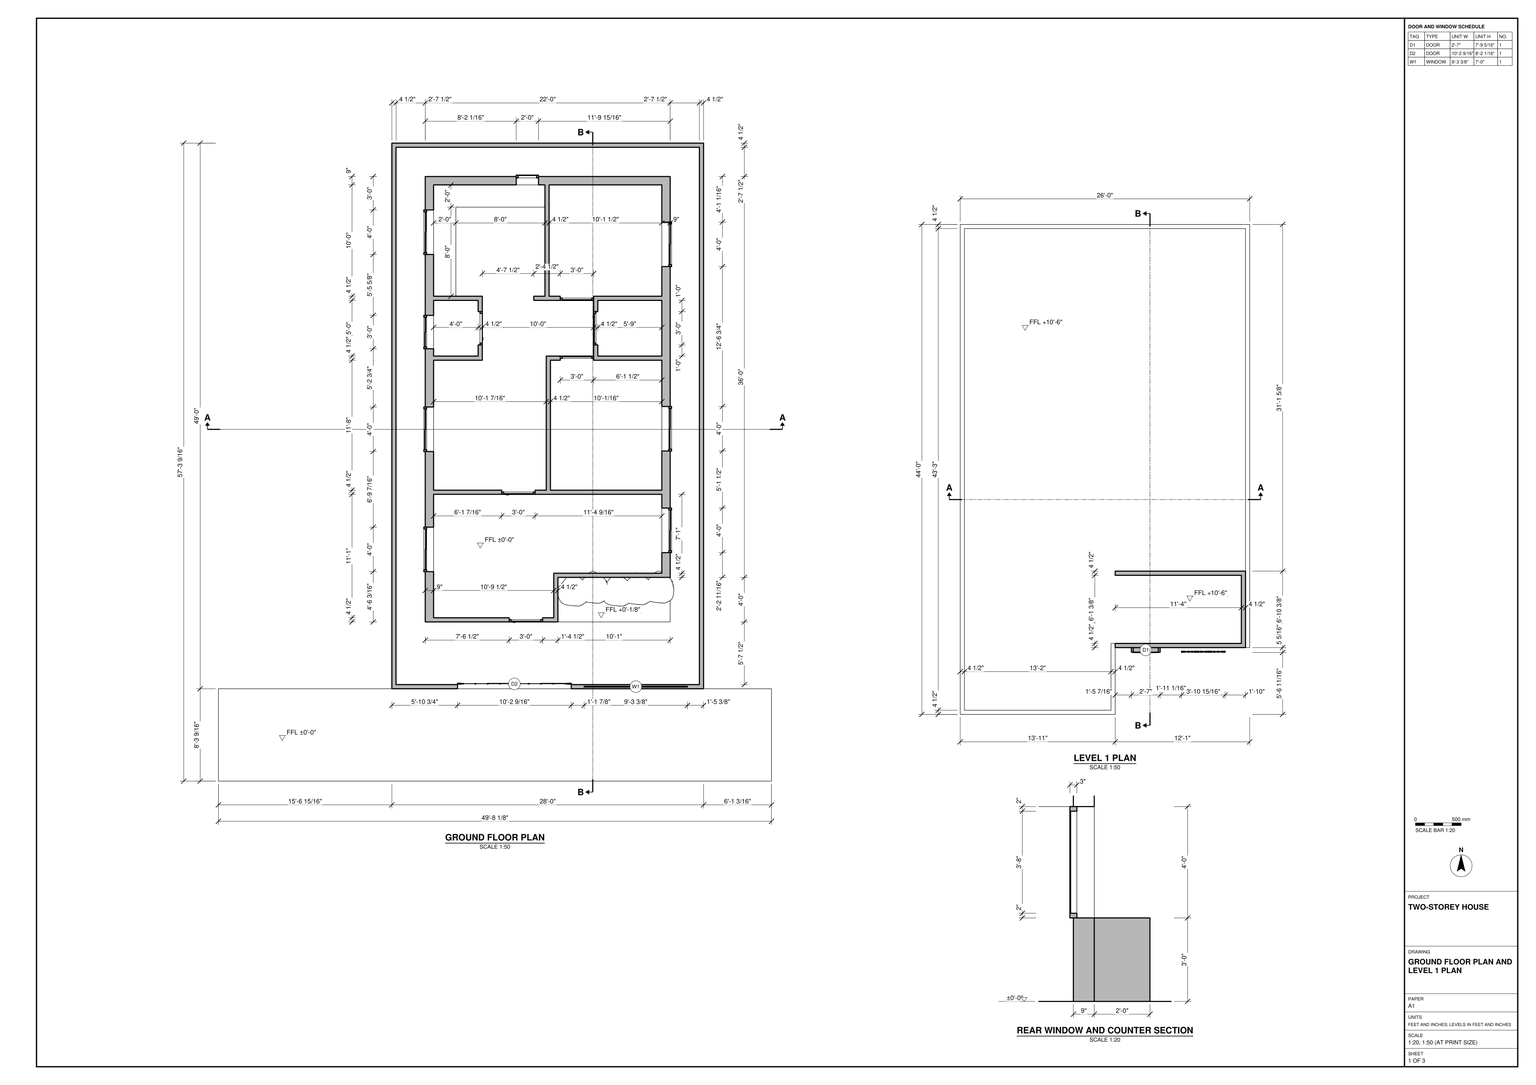
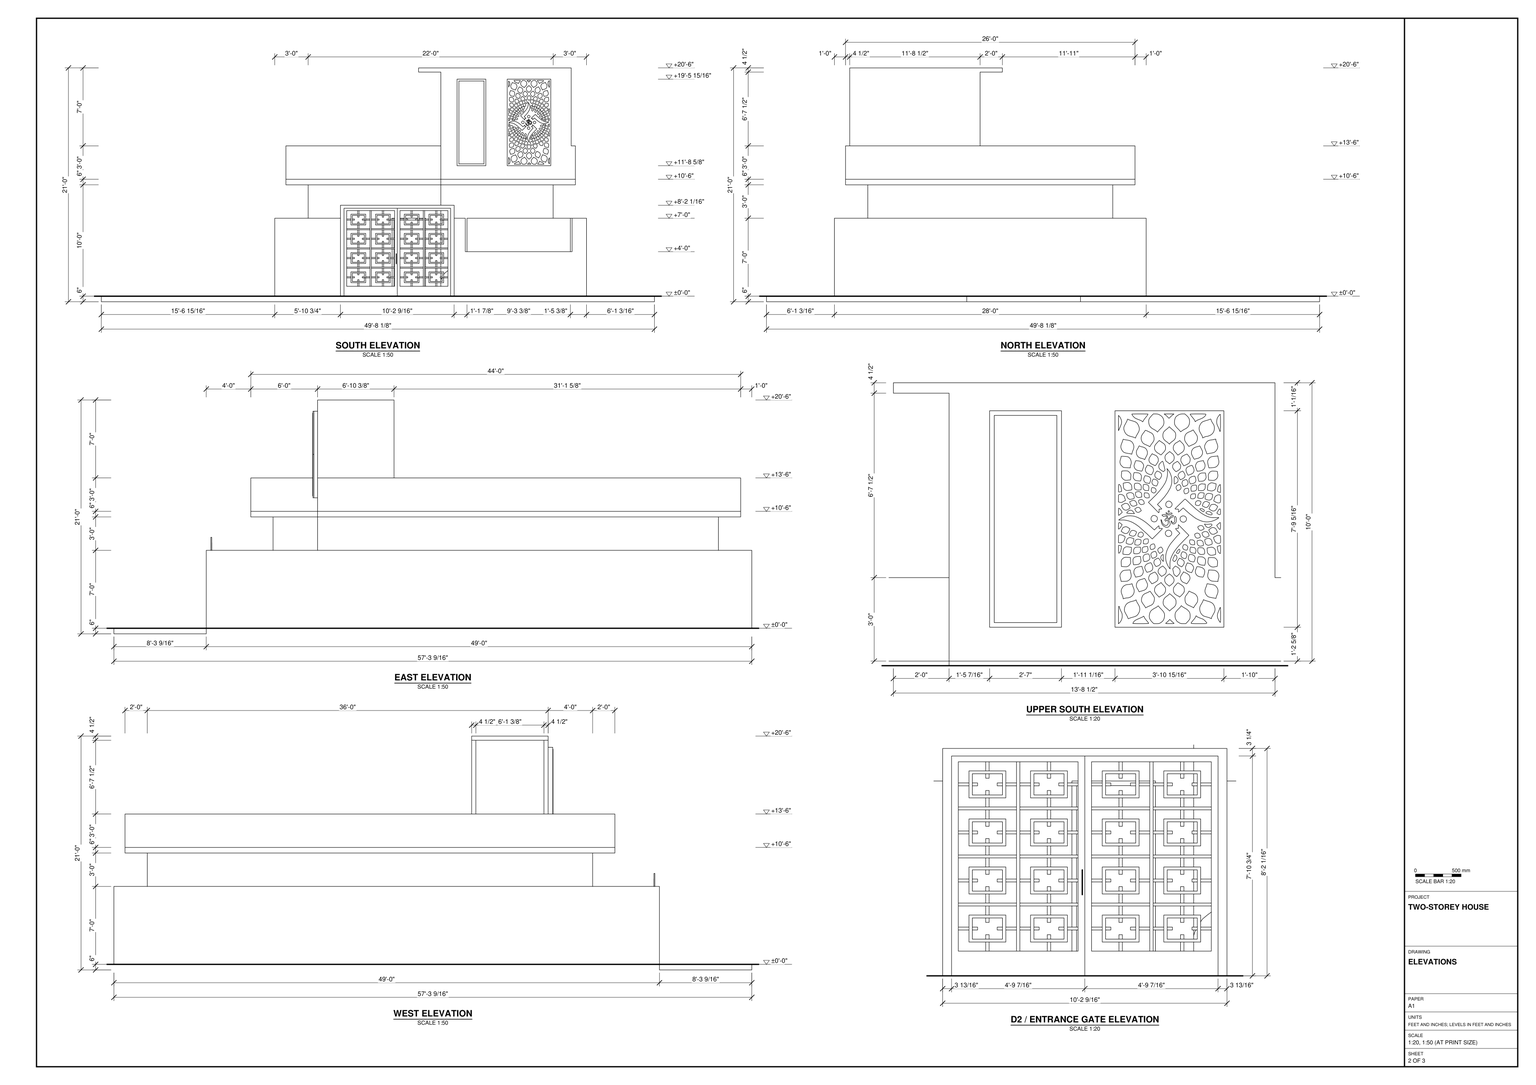
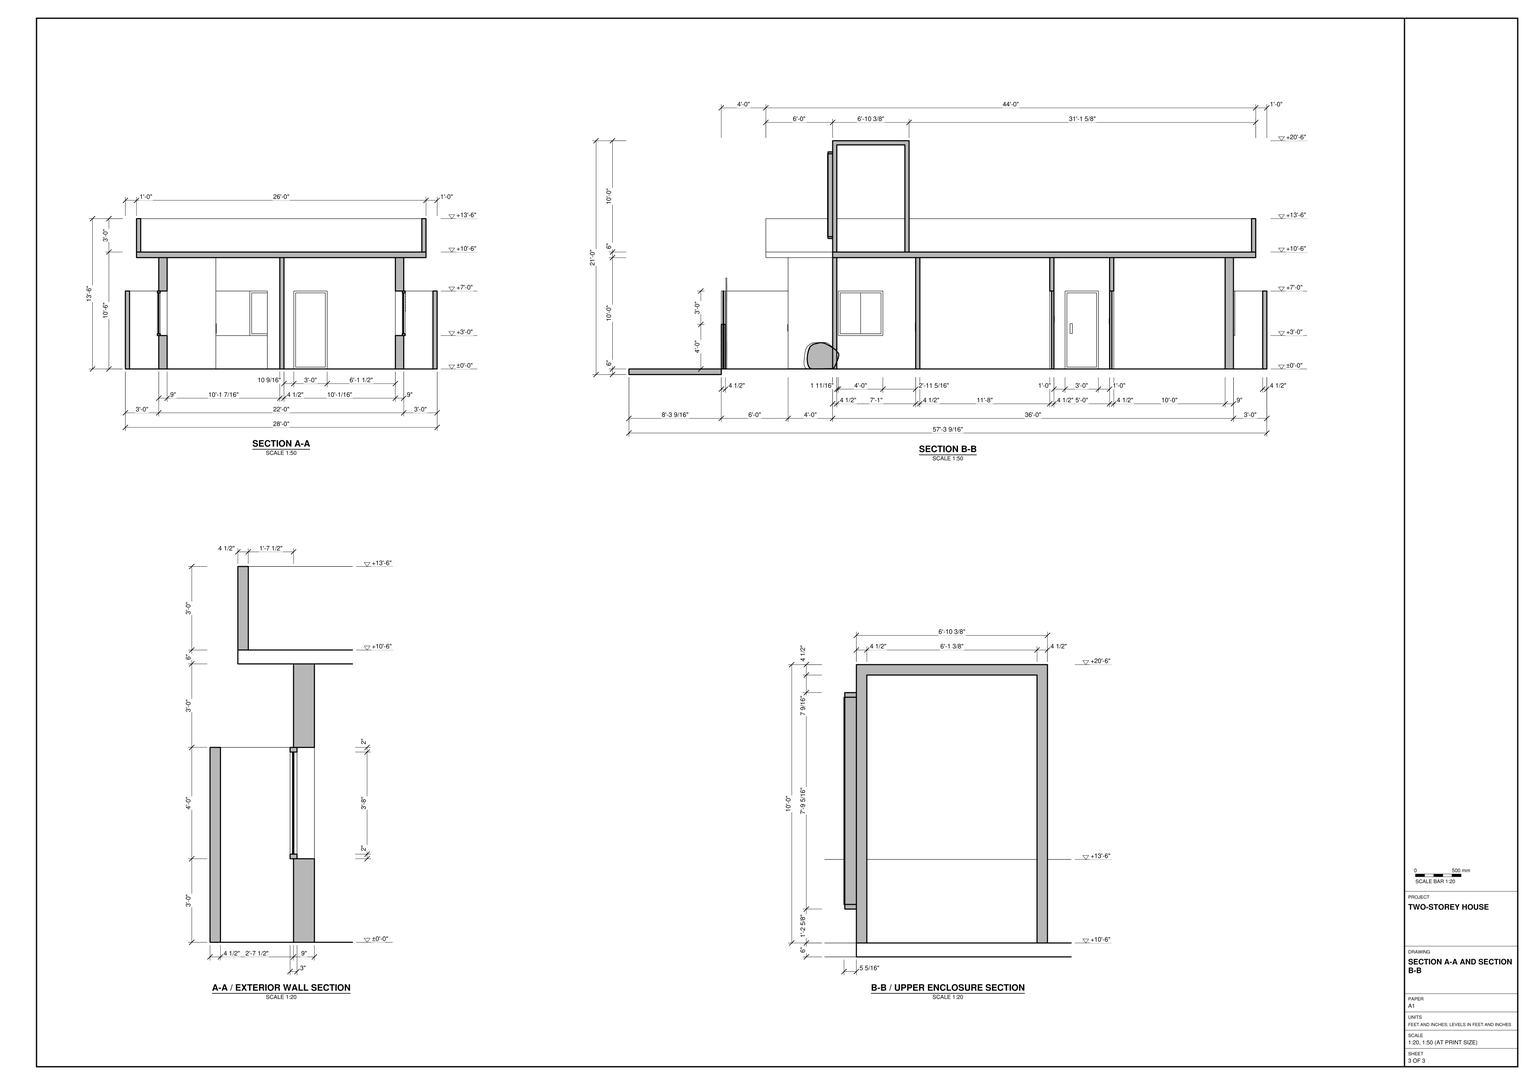
Build the house and its walled plot in SketchUp from task_files/diagram_01.pdf. Work in feet and inches. Including the apron outside the entrance, the model measures 49'-8 1/8" east to west, 57'-3 9/16" north to south and 21'-0" in overall height. Set the ground floor at ±0'-0" and the terrace floor at +10'-6".

Use the ground-floor plan to place the house inside the perimeter wall. Reproduce the stepped south end, the room divisions and the door and window openings. Distinguish the 9" exterior house walls from the 4 1/2" partitions. Fit the rear corner counter beneath the windows, using the counter section for its depth and height. On the south boundary, place the patterned double-leaf gate to the left of the wide window opening.

Model the projecting terrace slab, its stepped front edge and its low parapet. Keep most of the terrace open, with the small flat-roofed enclosure at the southeast end. Use the enlarged south elevation to position the enclosure door and the adjacent patterned panel.

Keep walls, slabs and roofs as separate groups or components, and group each furniture or joinery piece separately. Use components for repeated parts. Decor and loose items may be represented by any suitable library components. Save one SketchUp model as output_files/two_storey_house_with_a_gated_entrance_and_roof_terrace.skp.

# SketchUp Ruby script. Lengths in inches.
U = 1.inch
M = Sketchup.active_model
def pt(a) = Geom::Point3d.new(a.map { |v| v * U })
def face(e, loops, mat)
  f = e.add_face(loops[0].map { |a| pt(a) })
  loops[1..].each { |l| e.add_face(l.map { |a| pt(a) }).erase! }
  f.material = f.back_material = mat if mat
  f
end
# faces: each face lists its corners as indices into pts; further lists are holes
def faces(e, pts, list, mat = nil) = list.each { |f| face(e, (f[0].is_a?(Array) ? f : [f]).map { |l| l.map { |i| pts[i] } }, mat) }
# xy, xz, yz: faces in a plane at the given z, y or x. An outline is a flat list of corners, or four numbers for a rectangle; further outlines are holes
def ring(l) = l.size == 4 ? [[l[0], l[1]], [l[2], l[1]], [l[2], l[3]], [l[0], l[3]]] : l.each_slice(2).to_a
def flat(e, list, mat, &to3) = list.each { |f| face(e, (f[0].is_a?(Array) ? f : [f]).map { |l| ring(l).map { |u, v| to3.(u, v) } }, mat) }
def xy(e, z, list, mat = nil) = flat(e, list, mat) { |x, y| [x, y, z] }
def xz(e, y, list, mat = nil) = flat(e, list, mat) { |x, z| [x, y, z] }
def yz(e, x, list, mat = nil) = flat(e, list, mat) { |y, z| [x, y, z] }
def lines(e, pts, list) = list.each { |a, b| e.add_line(pt(pts[a]), pt(pts[b])) }
# prism: a flat outline (further loops are holes) pulled along v
def prism(e, loops, v, mat = nil)
  f = face(e, loops, mat); d = Geom::Vector3d.new(v.map { |x| x * U })
  f.pushpull(f.normal.samedirection?(d) ? d.length : -d.length)
end
def box(e, o, s, mat = nil) = prism(e, [[o, [o[0] + s[0], o[1], o[2]], [o[0] + s[0], o[1] + s[1], o[2]], [o[0], o[1] + s[1], o[2]]]], [0, 0, s[2]], mat)
def at(x, y, z, deg = 0) = Geom::Transformation.translation(pt([x, y, z])) * Geom::Transformation.rotation(ORIGIN, Z_AXIS, deg.degrees)
def axes(o, x, y, z) = Geom::Transformation.new([*x, 0, *y, 0, *z, 0, *pt(o).to_a, 1])
def part(name) = M.definitions.add(name)
# library, detail: a bought-in or finely detailed component or shape, given as its bounding box
def library(name, o, s) = part(name).tap { |d| box(d.entities, o, s) }
def detail(e, o, s) = box(e.add_group.entities, o, s)
def put(e, d, t, mat = nil) = e.add_instance(d, t).tap { |i| i.material = mat if mat }
def group(e, t, mat = nil) = e.add_group.tap { |g| g.transformation = t; g.material = mat if mat }.entities
root = M.entities
M.materials.add("Asphalt Black 15-01 100cm").color = [65, 65, 69]
M.materials.add("Glass Safety Frosted Rough 001").color = [38, 38, 38]
M.materials["Glass Safety Frosted Rough 001"].alpha = 0.1
M.materials.add("Grass D 200cm").color = [113, 140, 74]
M.materials.add("Metal Patina 002 180cm").color = [117, 110, 95]
M.materials.add("Onyx 100cm").color = [192, 149, 115]
M.materials.add("Roof Ceramic 22-10 200cm").color = [102, 65, 42]
M.materials.add("Tiles K01 100cm").color = [149, 135, 123]
M.materials.add("Wall Paint Bumpy 01 Blue 100cm").color = [86, 103, 109]
M.materials.add("Wall Paint Fine Grain 01 Yellow 100cm").color = [207, 190, 139]
M.materials.add("Wenge Highgloss 300cm").color = [70, 42, 26]
c1 = library("Skimmia japonica Rubella 004",[-17.08,-16.64,-0.26],[33.2,34.59,28.81])
c2 = library("gate 160k",[0,0,0],[125.98,5.98,118.11])
c3 = library("Dome Light",[-12,-12,0],[24,24,12])
c4 = part("Group\#23")
box(c4.entities,[-0.31,0,0],[0.31,22,44])
c5 = part("Group\#25")
box(c5.entities,[0,0,0],[0.31,20,2])
c6 = part("Group\#27")
box(c6.entities,[-0.31,0,0],[0.31,22,44])
c7 = part("Group\#31")
box(c7.entities,[0,0,0],[0.31,22,44])
c8 = part("Group\#33")
box(c8.entities,[0,0,0],[0.31,16,44])
c9 = part("Group\#35")
box(c9.entities,[0,0,0],[0.31,22,44])
c10 = part("Group\#37")
box(c10.entities,[0,0,0],[0.31,22,44])
c11 = part("Group\#21")
box(c11.entities,[-0.31,0,0],[0.31,22,44])
c12 = library("Group\#44",[0,0,0],[332.61,663.67,3])
xy(root,0,[[186.9375,99.5625,257.72,99.5625,257.72,104.0625,191.4375,104.0625,191.4375,683.0625,518.4375,683.0625,518.4375,104.0625,380.28,104.0625,380.28,99.5625,522.9375,99.5625,522.9375,687.5625,186.9375,687.5625]])
xy(root,0,[[257.72,99.5625,380.28,99.5625,380.28,104.0625,518.4375,104.0625,518.4375,683.0625,191.4375,683.0625,191.4375,104.0625,257.72,104.0625]],"Tiles K01 100cm")
xy(root,48,[[392.28,99.5625,507.41,104.0625]],"Wall Paint Fine Grain 01 Yellow 100cm")
xy(root,84,[[186.9375,99.5625,257.72,99.5625,257.72,104.0625,191.4375,104.0625,191.4375,683.0625,518.4375,683.0625,518.4375,104.0625,507.41,104.0625,507.41,99.5625,522.9375,99.5625,522.9375,687.5625,186.9375,687.5625],[380.28,99.5625,392.28,104.0625]],"Wall Paint Fine Grain 01 Yellow 100cm")
xz(root,99.5625,[[186.9375,0,257.72,84],[380.28,0,522.9375,0,522.9375,84,507.41,84,507.41,48,392.28,48,392.28,84,380.28,84]],"Wall Paint Fine Grain 01 Yellow 100cm")
xz(root,104.0625,[[191.4375,0,257.72,84],[380.28,0,380.28,84,392.28,84,392.28,48,507.41,48,507.41,84,518.4375,84,518.4375,0]],"Wall Paint Fine Grain 01 Yellow 100cm")
xz(root,683.0625,[[191.4375,0,518.4375,84]],"Wall Paint Fine Grain 01 Yellow 100cm")
xz(root,687.5625,[[186.9375,0,522.9375,84]],"Wall Paint Fine Grain 01 Yellow 100cm")
yz(root,186.9375,[[99.5625,0,687.5625,84]],"Wall Paint Fine Grain 01 Yellow 100cm")
yz(root,191.4375,[[104.0625,0,683.0625,84]],"Wall Paint Fine Grain 01 Yellow 100cm")
yz(root,257.72,[[99.5625,0,104.0625,84]],"Wall Paint Fine Grain 01 Yellow 100cm")
yz(root,380.28,[[99.5625,0,104.0625,84]],"Wall Paint Fine Grain 01 Yellow 100cm")
yz(root,392.28,[[99.5625,48,104.0625,84]],"Wall Paint Fine Grain 01 Yellow 100cm")
yz(root,507.41,[[99.5625,48,104.0625,84]],"Wall Paint Fine Grain 01 Yellow 100cm")
yz(root,518.4375,[[104.0625,0,683.0625,84]],"Wall Paint Fine Grain 01 Yellow 100cm")
yz(root,522.9375,[[99.5625,0,687.5625,84]],"Wall Paint Fine Grain 01 Yellow 100cm")
put(root,c1,at(382.15,205.3,0.1))
put(root,c1,at(403.95,208.32,0.1))
put(root,c1,at(429.53,205.21,0.1))
put(root,c1,at(451.61,206.6875,0.1))
put(root,c1,at(474.74,208.5,0.1))
put(root,c2,axes([257.72,104.0625,0],[0.97284,0,0],[0,0.24787,0],[0,0,0.83]))
put(root,c3,at(144.45,99.5625,25.05))
g1 = group(root,at(222.9375,171.5625,0))
xy(g1,0,[[0,0,0,480,264,480,264,48,143,48,143,0,126.5,0,126.5,4.5,138.5,4.5,138.5,52.5,255,52.5,255,137.5,118.4375,137.5,118.4375,142,130.4375,142,130.4375,286.5,145.5,286.5,145.5,282,134.9375,282,134.9375,142,255,142,255,282,181.5,282,181.5,298.5,186,298.5,186,286.5,255,286.5,255,346.5,186,346.5,186,334.5,181.5,334.5,181.5,351,255,351,255,471,133.5,471,133.5,351,145.5,351,145.5,346.5,117,346.5,117,351,129,351,129,471,9,471,9,351,61.5,351,61.5,334.5,57,334.5,57,346.5,9,346.5,9,286.5,57,286.5,57,298.5,61.5,298.5,61.5,282,9,282,9,142,82.4375,142,82.4375,137.5,9,137.5,9,4.5,90.5,4.5,90.5,0]])
xy(g1,36,[[0,54.16,9,102.16],[255,74.6875,264,122.6875],[0,183.62,9,231.62],[255,184.1875,264,232.1875],[0,294.37,9,330.37],
  [9,351,33,351,33,447,129,447,129,471,9,471],[255,382.9375,264,430.9375],[0,396,9,444],[98.0625,471,122.0625,480]])
xy(g1,60,[[255,298.75,264,322.75]])
xy(g1,84,[[90.5,0,126.5,4.5],[0,54.16,9,102.16],[255,74.6875,264,122.6875],[82.4375,137.5,118.4375,142],[0,183.62,9,231.62],
  [255,184.1875,264,232.1875],[145.5,282,181.5,286.5],[0,294.37,9,330.37],[57,298.5,61.5,334.5],[181.5,298.5,186,334.5],
  [255,298.75,264,322.75],[61.5,346.5,117,351],[145.5,346.5,181.5,351],[255,382.9375,264,430.9375],[0,396,9,444],
  [98.0625,471,122.0625,480]])
xy(g1,120,[[[0,0,143,0,143,48,264,48,264,480,0,480],[9,4.5,9,137.5,255,137.5,255,52.5,138.5,52.5,138.5,4.5],[9,142,9,282,61.5,282,61.5,346.5,181.5,346.5,181.5,286.5,130.4375,286.5,130.4375,142],[134.9375,142,255,282],[133.5,351,255,471],[9,351,129,471],[186,286.5,255,346.5],[9,286.5,57,346.5]]])
xz(g1,0,[[0,0,90.5,0,90.5,84,126.5,84,126.5,0,143,0,143,120,0,120]],"Wall Paint Bumpy 01 Blue 100cm")
xz(g1,4.5,[[9,0,9,120,138.5,120,138.5,0,126.5,0,126.5,84,90.5,84,90.5,0]])
xz(g1,48,[[143,0,264,120]],"Wall Paint Bumpy 01 Blue 100cm")
xz(g1,52.5,[[138.5,0,255,120]])
xz(g1,54.16,[[0,36,9,84]])
xz(g1,74.6875,[[255,36,264,84]])
xz(g1,102.16,[[0,36,9,84]])
xz(g1,122.6875,[[255,36,264,84]])
xz(g1,137.5,[[9,0,82.4375,0,82.4375,84,118.4375,84,118.4375,0,255,0,255,120,9,120]])
xz(g1,142,[[9,0,9,120,130.4375,120,130.4375,0,118.4375,0,118.4375,84,82.4375,84,82.4375,0],[134.9375,0,255,120]])
xz(g1,183.62,[[0,36,9,84]])
xz(g1,184.1875,[[255,36,264,84]])
xz(g1,231.62,[[0,36,9,84]])
xz(g1,232.1875,[[255,36,264,84]])
xz(g1,282,[[9,0,61.5,120],[134.9375,0,145.5,0,145.5,84,181.5,84,181.5,0,255,0,255,120,134.9375,120]])
xz(g1,286.5,[[9,0,57,120],[130.4375,0,130.4375,120,181.5,120,181.5,84,145.5,84,145.5,0],[186,0,255,120]])
xz(g1,294.37,[[0,36,9,84]])
xz(g1,298.5,[[57,0,61.5,84],[181.5,0,186,84]])
xz(g1,298.75,[[255,60,264,84]])
xz(g1,322.75,[[255,60,264,84]])
xz(g1,330.37,[[0,36,9,84]])
xz(g1,334.5,[[57,0,61.5,84],[181.5,0,186,84]])
xz(g1,346.5,[[9,0,57,120],[117,0,145.5,0,145.5,84,181.5,84,181.5,120,61.5,120,61.5,84,117,84],[186,0,255,120]])
xz(g1,351,[[33,0,33,36,9,36,9,120,61.5,120,61.5,0],[9,0,33,36],[117,0,117,84,61.5,84,61.5,120,129,120,129,0],[133.5,0,133.5,120,255,120,255,0,181.5,0,181.5,84,145.5,84,145.5,0]])
xz(g1,382.9375,[[255,36,264,84]])
xz(g1,396,[[0,36,9,84]])
xz(g1,430.9375,[[255,36,264,84]])
xz(g1,444,[[0,36,9,84]])
xz(g1,447,[[33,0,129,36]])
xz(g1,471,[[9,0,129,36],[133.5,0,255,120],[9,36,98.0625,36,98.0625,84,122.0625,84,122.0625,36,129,36,129,120,9,120]])
xz(g1,480,[[[0,0,264,120],[98.0625,36,122.0625,84]]],"Wall Paint Bumpy 01 Blue 100cm")
yz(g1,0,[[[0,0,480,120],[183.62,36,231.62,84],[54.16,36,102.16,84],[396,36,444,84],[294.37,36,330.37,84]]],"Wall Paint Bumpy 01 Blue 100cm")
yz(g1,9,[[[4.5,0,137.5,120],[54.16,36,102.16,84]],[[142,0,282,120],[183.62,36,231.62,84]],[[286.5,0,346.5,120],[294.37,36,330.37,84]],[351,0,471,36],[351,36,396,36,396,84,444,84,444,36,471,36,471,120,351,120]])
yz(g1,33,[[351,0,447,36]])
yz(g1,57,[[286.5,0,286.5,120,346.5,120,346.5,0,334.5,0,334.5,84,298.5,84,298.5,0]])
yz(g1,61.5,[[282,0,298.5,0,298.5,84,334.5,84,334.5,0,351,0,351,84,346.5,84,346.5,120,282,120]])
yz(g1,82.4375,[[137.5,0,142,84]])
yz(g1,90.5,[[0,0,4.5,84]])
yz(g1,98.0625,[[471,36,480,84]])
yz(g1,117,[[346.5,0,351,84]])
yz(g1,118.4375,[[137.5,0,142,84]])
yz(g1,122.0625,[[471,36,480,84]])
yz(g1,126.5,[[0,0,4.5,84]])
yz(g1,129,[[351,0,351,120,471,120,471,36,447,36,447,0],[447,0,471,36]])
yz(g1,130.4375,[[142,0,286.5,120]])
yz(g1,133.5,[[351,0,471,120]])
yz(g1,134.9375,[[142,0,282,120]])
yz(g1,138.5,[[4.5,0,52.5,120]])
yz(g1,143,[[0,0,48,120]],"Wall Paint Bumpy 01 Blue 100cm")
yz(g1,145.5,[[282,0,286.5,84],[346.5,0,351,84]])
yz(g1,181.5,[[282,0,286.5,84],[286.5,0,286.5,120,346.5,120,346.5,0,334.5,0,334.5,84,298.5,84,298.5,0],[346.5,0,351,84]])
yz(g1,186,[[286.5,0,298.5,0,298.5,84,334.5,84,334.5,0,346.5,0,346.5,120,286.5,120]])
yz(g1,255,[[[52.5,0,137.5,120],[74.6875,36,122.6875,84]],[[142,0,282,120],[184.1875,36,232.1875,84]],[[286.5,0,346.5,120],[298.75,60,322.75,84]],[[351,0,471,120],[382.9375,36,430.9375,84]]])
yz(g1,264,[[[48,0,480,120],[74.6875,36,122.6875,84],[184.1875,36,232.1875,84],[382.9375,36,430.9375,84],[298.75,60,322.75,84]]],"Wall Paint Bumpy 01 Blue 100cm")
p = [[90.5,0,0],[126.5,0,0],[82.4375,137.5,0],[118.4375,137.5,0],[61.5,298.5,0],[61.5,334.5,0],
  [181.5,334.5,0],[181.5,298.5,0],[181.5,286.5,0],[145.5,286.5,0],[145.5,346.5,0],[181.5,346.5,0]]
lines(g1,p,[[0,1],[2,3],[4,5],[6,7],[8,9],[10,11]])
g2 = group(g1,at(90.5,0,0))
prism(g2,[[[36,0,0],[36,0,84],[0,0,84],[0,0,0]],[[34,0,82],[34,0,2],[2,0,2],[2,0,82]]],[0,2.5,0],"Metal Patina 002 180cm")
g3 = group(g2,at(2,0,2))
box(g3,[0,0,0],[32,0.71,80],"Wenge Highgloss 300cm")
g4 = group(g3,at(2.54,0,38.66),"Metal Patina 002 180cm")
xy(g4,0,[[0,-0.5,1.5,0]])
xy(g4,7.25,[[0,-0.5,1.5,0]])
xz(g4,-0.5,[[0,0,1.5,7.25]],"Metal Patina 002 180cm")
xz(g4,0,[[0,0,1.5,7.25]],"Metal Patina 002 180cm")
yz(g4,0,[[-0.5,0,0,7.25]])
yz(g4,1.5,[[-0.5,0,0,7.25]])
g5 = group(g1,at(82.4375,137.5,0))
xy(g5,0,[[0,0,36,2.5]])
xy(g5,2,[[2,0,34,2.5]])
xy(g5,82,[[2,0,34,2.5]])
xy(g5,84,[[0,0,36,2.5]])
xz(g5,0,[[[0,0,36,84],[2,2,34,82]]],"Metal Patina 002 180cm")
xz(g5,2.5,[[[0,0,36,84],[2,2,34,82]]])
yz(g5,0,[[0,0,2.5,84]])
yz(g5,2,[[0,2,2.5,82]])
yz(g5,34,[[0,2,2.5,82]])
yz(g5,36,[[0,0,2.5,84]])
g6 = group(g5,at(2,0,2))
box(g6,[0,0,0],[32,0.71,80],"Wenge Highgloss 300cm")
g7 = group(g6,at(2.99,0,38.56),"Metal Patina 002 180cm")
xy(g7,0,[[0,-0.5,2.1875,0]])
xy(g7,9.3125,[[0,-0.5,2.1875,0]])
xz(g7,-0.5,[[0,0,2.1875,9.3125]],"Metal Patina 002 180cm")
xz(g7,0,[[0,0,2.1875,9.3125]],"Metal Patina 002 180cm")
yz(g7,0,[[-0.5,0,0,9.3125]])
yz(g7,2.1875,[[-0.5,0,0,9.3125]])
g8 = group(g1,at(61.5,298.5,0))
prism(g8,[[[0,36,0],[0,36,84],[0,0,84],[0,0,0]],[[0,34,82],[0,34,2],[0,2,2],[0,2,82]]],[-2.5,0,0],"Metal Patina 002 180cm")
g9 = group(g8,at(0,2,2),"Wenge Highgloss 300cm")
yz(g9,0,[[0,0,32,80]],"Wenge Highgloss 300cm")
g10 = group(g8,at(0,5.36,38.26),"Metal Patina 002 180cm")
xy(g10,0,[[0,0,0.5,2.54]])
xy(g10,10.59,[[0,0,0.5,2.54]])
xz(g10,0,[[0,0,0.5,10.59]],"Metal Patina 002 180cm")
xz(g10,2.54,[[0,0,0.5,10.59]],"Metal Patina 002 180cm")
yz(g10,0,[[0,0,2.54,10.59]],"Metal Patina 002 180cm")
yz(g10,0.5,[[0,0,2.54,10.59]],"Metal Patina 002 180cm")
g11 = group(g1,at(181.5,298.5,0))
prism(g11,[[[0,0,0],[0,0,84],[0,36,84],[0,36,0]],[[0,34,82],[0,2,82],[0,2,2],[0,34,2]]],[2.5,0,0],"Metal Patina 002 180cm")
g12 = group(g11,at(0,2,2))
box(g12,[0,0,0],[0.71,32,80],"Wenge Highgloss 300cm")
g13 = group(g12,at(0,28.62,41.48),"Metal Patina 002 180cm")
xy(g13,0,[[-0.5,-1.1875,0,0]])
xy(g13,6.8125,[[-0.5,-1.1875,0,0]])
xz(g13,-1.1875,[[-0.5,0,0,6.8125]])
xz(g13,0,[[-0.5,0,0,6.8125]])
yz(g13,-0.5,[[-1.1875,0,0,6.8125]],"Metal Patina 002 180cm")
yz(g13,0,[[-1.1875,0,0,6.8125]],"Metal Patina 002 180cm")
g14 = group(g1,at(145.5,286.5,0))
xy(g14,0,[[0,-2.5,36,0]])
xy(g14,2,[[2,-2.5,34,0]])
xy(g14,82,[[2,-2.5,34,0]])
xy(g14,84,[[0,-2.5,36,0]])
xz(g14,-2.5,[[[0,0,36,84],[2,2,34,82]]])
xz(g14,0,[[[0,0,36,84],[2,2,34,82]]],"Metal Patina 002 180cm")
yz(g14,0,[[-2.5,0,0,84]])
yz(g14,2,[[-2.5,2,0,82]])
yz(g14,34,[[-2.5,2,0,82]])
yz(g14,36,[[-2.5,0,0,84]])
g15 = group(g14,at(2,0,2))
box(g15,[0,-0.71,0],[32,0.71,80],"Wenge Highgloss 300cm")
g16 = group(g15,at(27.97,0,48.31),"Metal Patina 002 180cm")
xy(g16,0,[[-1.25,0,0,0.5]])
xy(g16,6.8125,[[-1.25,0,0,0.5]])
xz(g16,0,[[-1.25,0,0,6.8125]],"Metal Patina 002 180cm")
xz(g16,0.5,[[-1.25,0,0,6.8125]],"Metal Patina 002 180cm")
yz(g16,-1.25,[[0,0,0.5,6.8125]])
yz(g16,0,[[0,0,0.5,6.8125]])
g17 = group(g1,at(145.5,346.5,0))
prism(g17,[[[36,0,0],[36,0,84],[0,0,84],[0,0,0]],[[34,0,2],[2,0,2],[2,0,82],[34,0,82]]],[0,2.5,0],"Metal Patina 002 180cm")
g18 = group(g17,at(2,0,2))
box(g18,[0,0,0],[32,0.71,80],"Wenge Highgloss 300cm")
g19 = group(g18,at(3.125,0,46.56),"Metal Patina 002 180cm")
xy(g19,0,[[0,-0.5,1.5,0]])
xy(g19,6.125,[[0,-0.5,1.5,0]])
xz(g19,-0.5,[[0,0,1.5,6.125]],"Metal Patina 002 180cm")
xz(g19,0,[[0,0,1.5,6.125]],"Metal Patina 002 180cm")
yz(g19,0,[[-0.5,0,0,6.125]])
yz(g19,1.5,[[-0.5,0,0,6.125]])
g20 = group(g1,at(264,184.1875,36))
xy(g20,0,[[-1.5,0,1.5,48]],"Metal Patina 002 180cm")
xy(g20,2,[[-1.5,2,1.5,46]],"Metal Patina 002 180cm")
xy(g20,46,[[-1.5,2,1.5,46]],"Metal Patina 002 180cm")
xy(g20,48,[[-1.5,0,1.5,48]],"Metal Patina 002 180cm")
xz(g20,0,[[-1.5,0,1.5,48]],"Metal Patina 002 180cm")
xz(g20,2,[[-1.5,2,1.5,46]],"Metal Patina 002 180cm")
xz(g20,46,[[-1.5,2,1.5,46]],"Metal Patina 002 180cm")
xz(g20,48,[[-1.5,0,1.5,48]],"Metal Patina 002 180cm")
yz(g20,-1.5,[[[0,0,48,48],[2,2,46,46]]],"Metal Patina 002 180cm")
yz(g20,1.5,[[[0,0,48,48],[2,2,46,46]]],"Metal Patina 002 180cm")
put(g20,c4,at(-0.3125,2,2),"Glass Safety Frosted Rough 001")
put(g20,c4,at(0,24,2),"Glass Safety Frosted Rough 001")
g21 = group(g1,at(264,298.75,60))
xy(g21,0,[[-1.5,0,1.5,24]],"Metal Patina 002 180cm")
xy(g21,2,[[-1.5,2,1.5,22]],"Metal Patina 002 180cm")
xy(g21,22,[[-1.5,2,1.5,22]],"Metal Patina 002 180cm")
xy(g21,24,[[-1.5,0,1.5,24]],"Metal Patina 002 180cm")
xz(g21,0,[[-1.5,0,1.5,24]],"Metal Patina 002 180cm")
xz(g21,2,[[-1.5,2,1.5,22]],"Metal Patina 002 180cm")
xz(g21,22,[[-1.5,2,1.5,22]],"Metal Patina 002 180cm")
xz(g21,24,[[-1.5,0,1.5,24]],"Metal Patina 002 180cm")
yz(g21,-1.5,[[[0,0,24,24],[2,2,22,22]]],"Metal Patina 002 180cm")
yz(g21,1.5,[[[0,0,24,24],[2,2,22,22]]],"Metal Patina 002 180cm")
put(g21,c5,at(1.5,2,20),"Glass Safety Frosted Rough 001")
put(g21,c5,at(1.5,2,17),"Glass Safety Frosted Rough 001")
put(g21,c5,at(1.5,2,14),"Glass Safety Frosted Rough 001")
put(g21,c5,at(1.5,2,11),"Glass Safety Frosted Rough 001")
put(g21,c5,at(1.5,2,8),"Glass Safety Frosted Rough 001")
put(g21,c5,at(1.5,2,5),"Glass Safety Frosted Rough 001")
put(g21,c5,at(1.5,2,2),"Glass Safety Frosted Rough 001")
g22 = group(g1,at(264,382.9375,36))
xy(g22,0,[[-1.5,0,1.5,48]],"Metal Patina 002 180cm")
xy(g22,2,[[-1.5,2,1.5,46]],"Metal Patina 002 180cm")
xy(g22,46,[[-1.5,2,1.5,46]],"Metal Patina 002 180cm")
xy(g22,48,[[-1.5,0,1.5,48]],"Metal Patina 002 180cm")
xz(g22,0,[[-1.5,0,1.5,48]],"Metal Patina 002 180cm")
xz(g22,2,[[-1.5,2,1.5,46]],"Metal Patina 002 180cm")
xz(g22,46,[[-1.5,2,1.5,46]],"Metal Patina 002 180cm")
xz(g22,48,[[-1.5,0,1.5,48]],"Metal Patina 002 180cm")
yz(g22,-1.5,[[[0,0,48,48],[2,2,46,46]]],"Metal Patina 002 180cm")
yz(g22,1.5,[[[0,0,48,48],[2,2,46,46]]],"Metal Patina 002 180cm")
put(g22,c6,at(-0.1875,2,2),"Glass Safety Frosted Rough 001")
put(g22,c6,at(0.13,24,2),"Glass Safety Frosted Rough 001")
g23 = group(g1,at(98.0625,480,36))
prism(g23,[[[24,1.5,0],[0,1.5,0],[0,1.5,48],[24,1.5,48]],[[22,1.5,2],[22,1.5,46],[2,1.5,46],[2,1.5,2]]],[0,-3,0],"Metal Patina 002 180cm")
g24 = group(g23,at(2,1.5,2),"Glass Safety Frosted Rough 001")
box(g24,[0,-0.31,0],[20,0.31,44])
g25 = group(g1,at(0,396,36))
xy(g25,0,[[-1.5,0,1.5,48]],"Metal Patina 002 180cm")
xy(g25,2,[[-1.5,2,1.5,46]],"Metal Patina 002 180cm")
xy(g25,46,[[-1.5,2,1.5,46]],"Metal Patina 002 180cm")
xy(g25,48,[[-1.5,0,1.5,48]],"Metal Patina 002 180cm")
xz(g25,0,[[-1.5,0,1.5,48]],"Metal Patina 002 180cm")
xz(g25,2,[[-1.5,2,1.5,46]],"Metal Patina 002 180cm")
xz(g25,46,[[-1.5,2,1.5,46]],"Metal Patina 002 180cm")
xz(g25,48,[[-1.5,0,1.5,48]],"Metal Patina 002 180cm")
yz(g25,-1.5,[[[0,0,48,48],[2,2,46,46]]],"Metal Patina 002 180cm")
yz(g25,1.5,[[[0,0,48,48],[2,2,46,46]]],"Metal Patina 002 180cm")
put(g25,c7,at(0.25,24,2),"Glass Safety Frosted Rough 001")
put(g25,c7,at(-0.06,2,2),"Glass Safety Frosted Rough 001")
g26 = group(g1,at(0,294.37,36))
xy(g26,0,[[-1.5,0,1.5,36]],"Metal Patina 002 180cm")
xy(g26,2,[[-1.5,2,1.5,34]],"Metal Patina 002 180cm")
xy(g26,46,[[-1.5,2,1.5,34]],"Metal Patina 002 180cm")
xy(g26,48,[[-1.5,0,1.5,36]],"Metal Patina 002 180cm")
xz(g26,0,[[-1.5,0,1.5,48]],"Metal Patina 002 180cm")
xz(g26,2,[[-1.5,2,1.5,46]],"Metal Patina 002 180cm")
xz(g26,34,[[-1.5,2,1.5,46]],"Metal Patina 002 180cm")
xz(g26,36,[[-1.5,0,1.5,48]],"Metal Patina 002 180cm")
yz(g26,-1.5,[[[0,0,36,48],[2,2,34,46]]],"Metal Patina 002 180cm")
yz(g26,1.5,[[[0,0,36,48],[2,2,34,46]]],"Metal Patina 002 180cm")
put(g26,c8,at(0,18,2),"Glass Safety Frosted Rough 001")
put(g26,c8,at(-0.31,2,2),"Glass Safety Frosted Rough 001")
g27 = group(g1,at(0,183.62,36))
xy(g27,0,[[-1.5,0,1.5,48]],"Metal Patina 002 180cm")
xy(g27,2,[[-1.5,2,1.5,46]],"Metal Patina 002 180cm")
xy(g27,46,[[-1.5,2,1.5,46]],"Metal Patina 002 180cm")
xy(g27,48,[[-1.5,0,1.5,48]],"Metal Patina 002 180cm")
xz(g27,0,[[-1.5,0,1.5,48]],"Metal Patina 002 180cm")
xz(g27,2,[[-1.5,2,1.5,46]],"Metal Patina 002 180cm")
xz(g27,46,[[-1.5,2,1.5,46]],"Metal Patina 002 180cm")
xz(g27,48,[[-1.5,0,1.5,48]],"Metal Patina 002 180cm")
yz(g27,-1.5,[[[0,0,48,48],[2,2,46,46]]],"Metal Patina 002 180cm")
yz(g27,1.5,[[[0,0,48,48],[2,2,46,46]]],"Metal Patina 002 180cm")
put(g27,c9,at(-0.0625,24,2),"Glass Safety Frosted Rough 001")
put(g27,c9,at(-0.38,2,2),"Glass Safety Frosted Rough 001")
g28 = group(g1,at(0,54.16,36))
xy(g28,0,[[-1.5,0,1.5,48]],"Metal Patina 002 180cm")
xy(g28,2,[[-1.5,2,1.5,46]],"Metal Patina 002 180cm")
xy(g28,46,[[-1.5,2,1.5,46]],"Metal Patina 002 180cm")
xy(g28,48,[[-1.5,0,1.5,48]],"Metal Patina 002 180cm")
xz(g28,0,[[-1.5,0,1.5,48]],"Metal Patina 002 180cm")
xz(g28,2,[[-1.5,2,1.5,46]],"Metal Patina 002 180cm")
xz(g28,46,[[-1.5,2,1.5,46]],"Metal Patina 002 180cm")
xz(g28,48,[[-1.5,0,1.5,48]],"Metal Patina 002 180cm")
yz(g28,-1.5,[[[0,0,48,48],[2,2,46,46]]],"Metal Patina 002 180cm")
yz(g28,1.5,[[[0,0,48,48],[2,2,46,46]]],"Metal Patina 002 180cm")
put(g28,c10,at(0.4375,24,2),"Glass Safety Frosted Rough 001")
put(g28,c10,at(0.12,2,2),"Glass Safety Frosted Rough 001")
g29 = group(g1,at(264,74.6875,36))
xy(g29,0,[[-1.5,0,1.5,48]],"Metal Patina 002 180cm")
xy(g29,2,[[-1.5,2,1.5,46]],"Metal Patina 002 180cm")
xy(g29,46,[[-1.5,2,1.5,46]],"Metal Patina 002 180cm")
xy(g29,48,[[-1.5,0,1.5,48]],"Metal Patina 002 180cm")
xz(g29,0,[[-1.5,0,1.5,48]],"Metal Patina 002 180cm")
xz(g29,2,[[-1.5,2,1.5,46]],"Metal Patina 002 180cm")
xz(g29,46,[[-1.5,2,1.5,46]],"Metal Patina 002 180cm")
xz(g29,48,[[-1.5,0,1.5,48]],"Metal Patina 002 180cm")
yz(g29,-1.5,[[[0,0,48,48],[2,2,46,46]]],"Metal Patina 002 180cm")
yz(g29,1.5,[[[0,0,48,48],[2,2,46,46]]],"Metal Patina 002 180cm")
put(g29,c11,at(0,2,2),"Glass Safety Frosted Rough 001")
put(g29,c11,at(0.3125,24,2),"Glass Safety Frosted Rough 001")
g30 = group(g1,at(143,0,0),"Grass D 200cm")
box(g30,[0,0,0],[121,48,0.1])
g31 = group(root,at(222.9375,219.5625,120))
xy(g31,0,[[-24,-72,-24,456,288,456,288,0,143,0,143,-72]],"Onyx 100cm")
xy(g31,6,[[-19.5,-67.5,138.5,-67.5,138.5,4.5,283.5,4.5,283.5,451.5,-19.5,451.5]])
xz(g31,-72,[[-24,0,143,6]],"Onyx 100cm")
xz(g31,0,[[143,0,288,6]],"Onyx 100cm")
xz(g31,456,[[-24,0,288,6]],"Onyx 100cm")
yz(g31,-24,[[-72,0,456,6]],"Onyx 100cm")
yz(g31,143,[[-72,0,0,6]],"Onyx 100cm")
yz(g31,288,[[0,0,456,6]],"Onyx 100cm")
g32 = group(g31,at(-24,-72,6),"Wall Paint Fine Grain 01 Yellow 100cm")
xy(g32,0,[[[0,0,0,528,312,528,312,72,167,72,167,0],[4.5,4.5,162.5,4.5,162.5,76.5,303,76.5,303,149.875,167,149.875,167,154.375,307.5,154.375,307.5,523.5,4.5,523.5]]],"Wall Paint Fine Grain 01 Yellow 100cm")
xy(g32,36,[[0,0,167,0,167,76.5,162.5,76.5,162.5,4.5,4.5,4.5,4.5,523.5,307.5,523.5,307.5,72,312,72,312,528,0,528]],"Wall Paint Fine Grain 01 Yellow 100cm")
xy(g32,115.5,[[143,72,167,76.5],[143,76.5,303,149.875],[143,149.875,167,154.375]],"Wall Paint Fine Grain 01 Yellow 100cm")
xy(g32,120,[[143,72,307.5,154.375]],"Wall Paint Fine Grain 01 Yellow 100cm")
xz(g32,0,[[0,0,167,36]],"Wall Paint Fine Grain 01 Yellow 100cm")
xz(g32,4.5,[[4.5,0,162.5,36]],"Wall Paint Fine Grain 01 Yellow 100cm")
xz(g32,72,[[167,0,312,0,312,36,307.5,36,307.5,120,143,120,143,115.5,167,115.5]],"Roof Ceramic 22-10 200cm")
xz(g32,76.5,[[162.5,0,162.5,36,167,36,167,115.5,303,115.5,303,0]],"Wall Paint Fine Grain 01 Yellow 100cm")
xz(g32,149.875,[[167,0,303,115.5]],"Wall Paint Fine Grain 01 Yellow 100cm")
xz(g32,154.375,[[167,0,167,115.5,143,115.5,143,120,307.5,120,307.5,0]],"Wall Paint Fine Grain 01 Yellow 100cm")
xz(g32,523.5,[[4.5,0,307.5,36]],"Wall Paint Fine Grain 01 Yellow 100cm")
xz(g32,528,[[0,0,312,36]],"Wall Paint Fine Grain 01 Yellow 100cm")
yz(g32,0,[[0,0,528,36]],"Wall Paint Fine Grain 01 Yellow 100cm")
yz(g32,4.5,[[4.5,0,523.5,36]],"Wall Paint Fine Grain 01 Yellow 100cm")
yz(g32,143,[[72,115.5,154.375,120]],"Wall Paint Fine Grain 01 Yellow 100cm")
yz(g32,162.5,[[4.5,0,76.5,36]],"Wall Paint Fine Grain 01 Yellow 100cm")
yz(g32,167,[[0,0,72,36],[149.875,0,154.375,115.5],[72,36,76.5,115.5]],"Wall Paint Fine Grain 01 Yellow 100cm")
yz(g32,303,[[76.5,0,149.875,115.5]],"Wall Paint Fine Grain 01 Yellow 100cm")
yz(g32,307.5,[[154.375,0,523.5,36],[72,36,154.375,120]],"Wall Paint Fine Grain 01 Yellow 100cm")
yz(g32,312,[[72,0,528,36]],"Wall Paint Fine Grain 01 Yellow 100cm")
g33 = group(g32,at(184.47,72,14.61),"Metal Patina 002 180cm")
prism(g33,[[[0,0,93.3125],[31,0,93.3125],[31,0,0],[0,0,0]],[[2,0,91.3125],[2,0,2],[29,0,2],[29,0,91.3125]]],[0,-5,0],"Metal Patina 002 180cm")
g34 = group(root,at(382.15,101.43,48),"Glass Safety Frosted Rough 001")
box(g34,[12,0,-48],[111.39,0.76,84],"Glass Safety Frosted Rough 001")
g35 = group(root,at(385.4,214.5625,142.61),"Glass Safety Frosted Rough 001")
box(g35,[0,-0.31,0],[27,0.31,89.3125])
put(root,c12,axes([437.47,215.64,140.61],[0.14115,0,0],[0,0,0.1406],[0,-0.36079,0]))
g36 = group(root,at(186.9375,50.3125,0),"Asphalt Black 15-01 100cm")
prism(g36,[[[-186.9375,49.25,-6],[70.78,49.25,-6],[193.34,49.25,-6],[409.1875,49.25,-6],[409.1875,-50.3125,-6],[-186.9375,-50.3125,-6]]],[0,0,6],"Asphalt Black 15-01 100cm")
